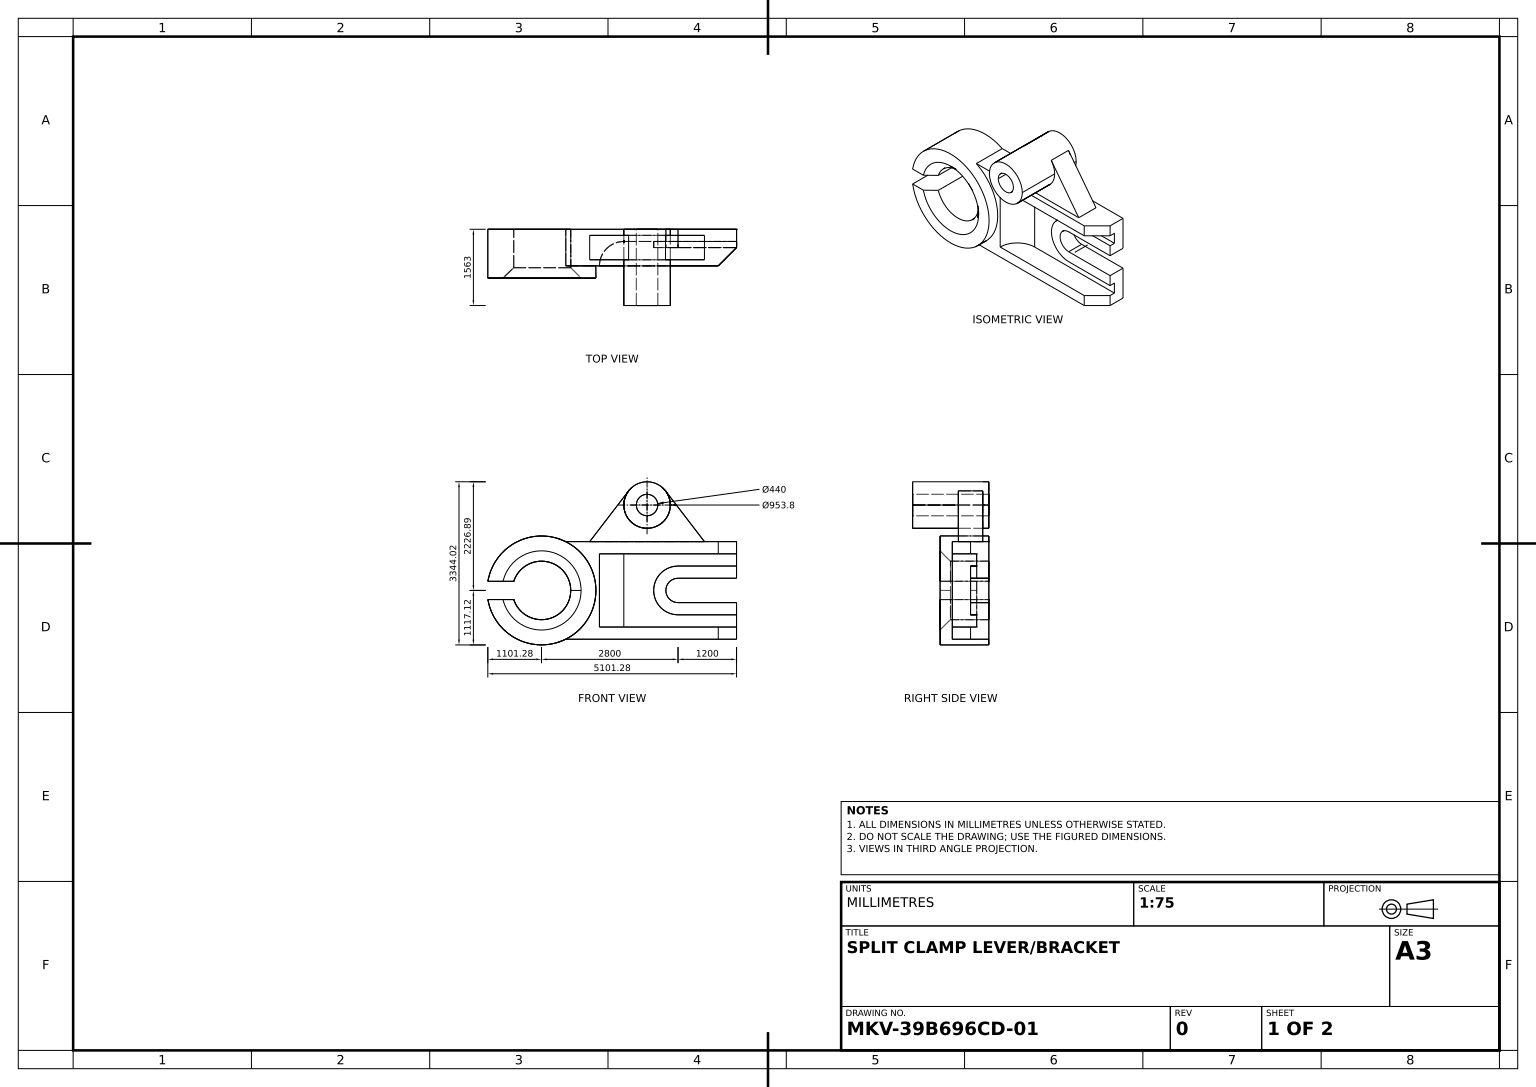
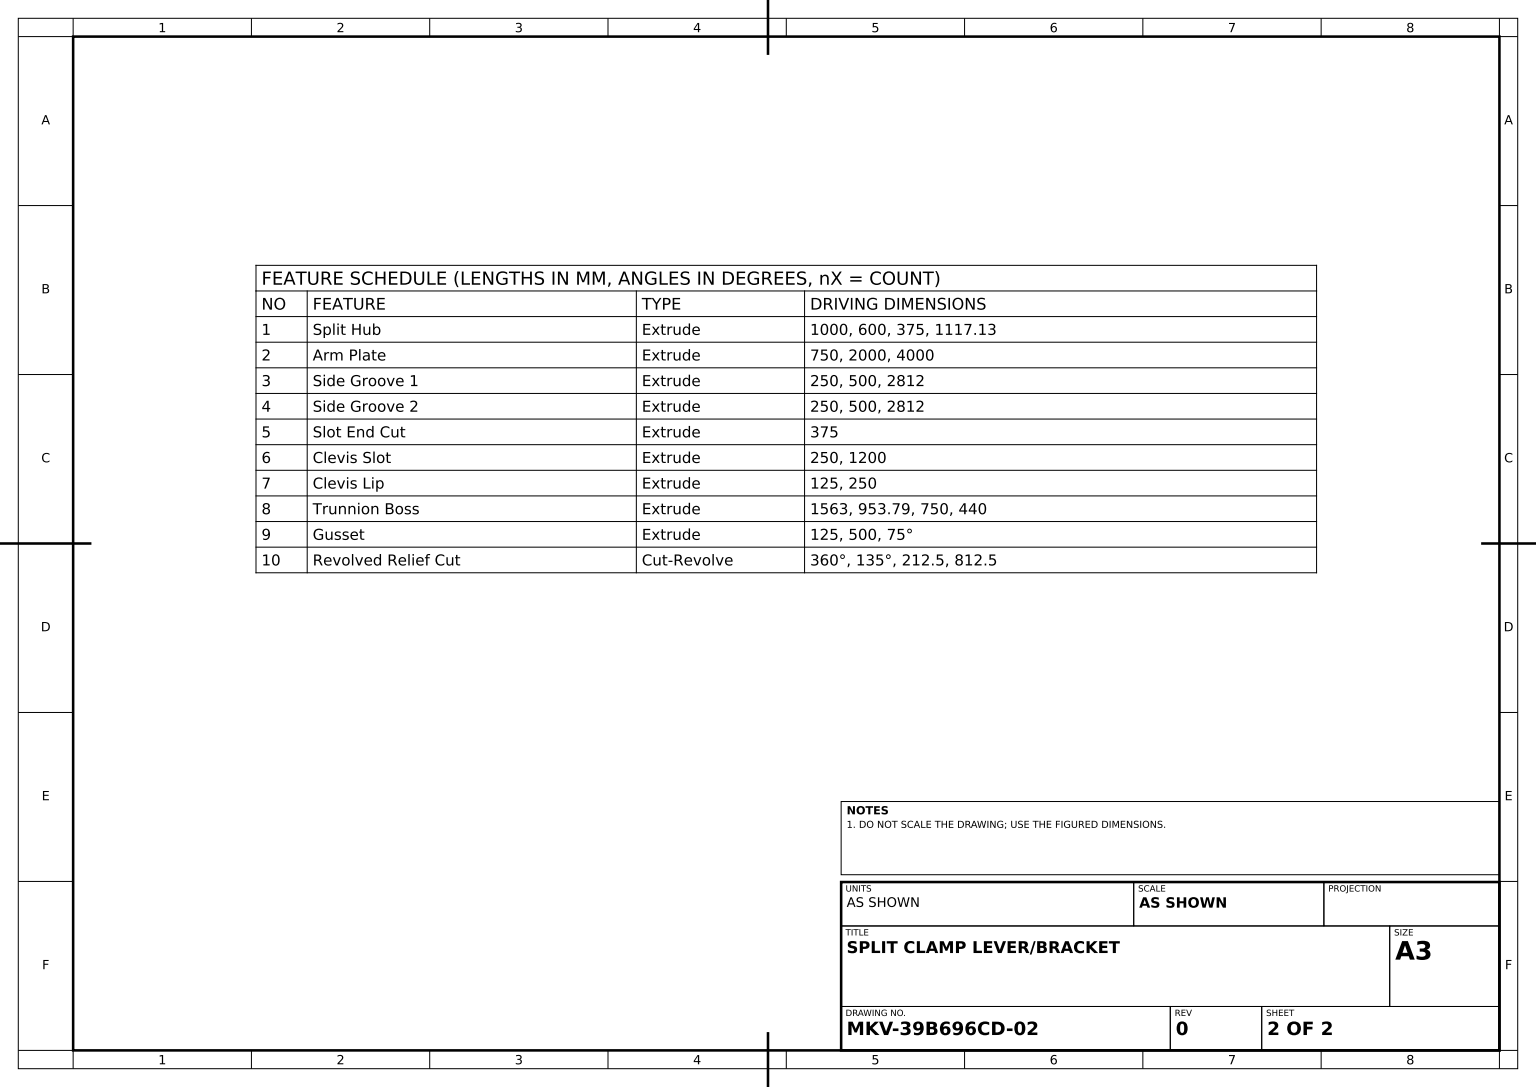
ISO-10303-21;
HEADER;
FILE_DESCRIPTION((''),'2;1');
FILE_NAME('','',(''),(''),'','','');
FILE_SCHEMA(('AUTOMOTIVE_DESIGN'));
ENDSEC;
DATA;
#1=APPLICATION_CONTEXT('');
#2=PRODUCT_CONTEXT('',#1,'mechanical');
#3=PRODUCT('','','',(#2));
#4=PRODUCT_DEFINITION_FORMATION('','',#3);
#5=PRODUCT_DEFINITION_CONTEXT('',#1,'design');
#6=PRODUCT_DEFINITION('','',#4,#5);
#7=PRODUCT_DEFINITION_SHAPE('','',#6);
#8=(LENGTH_UNIT()NAMED_UNIT(*)SI_UNIT(.MILLI.,.METRE.));
#9=(NAMED_UNIT(*)PLANE_ANGLE_UNIT()SI_UNIT($,.RADIAN.));
#10=(NAMED_UNIT(*)SI_UNIT($,.STERADIAN.)SOLID_ANGLE_UNIT());
#11=UNCERTAINTY_MEASURE_WITH_UNIT(LENGTH_MEASURE(1.E-05),#8,'distance_accuracy_value','');
#12=(GEOMETRIC_REPRESENTATION_CONTEXT(3)GLOBAL_UNCERTAINTY_ASSIGNED_CONTEXT((#11))GLOBAL_UNIT_ASSIGNED_CONTEXT((#8,#9,#10))REPRESENTATION_CONTEXT('',''));
#13=CARTESIAN_POINT('',(4000.,750.,250.));
#14=VERTEX_POINT('',#13);
#15=CARTESIAN_POINT('',(4000.,750.,375.));
#16=VERTEX_POINT('',#15);
#17=CARTESIAN_POINT('',(4000.,750.,750.));
#18=DIRECTION('',(0.,0.,1.));
#19=VECTOR('',#18,1000.);
#20=LINE('',#17,#19);
#21=EDGE_CURVE('',#14,#16,#20,.T.);
#22=ORIENTED_EDGE('',*,*,#21,.F.);
#23=CARTESIAN_POINT('',(4000.,500.,250.));
#24=VERTEX_POINT('',#23);
#25=CARTESIAN_POINT('',(4000.,3856.106441,250.));
#26=DIRECTION('',(0.,-1.,0.));
#27=VECTOR('',#26,1000.);
#28=LINE('',#25,#27);
#29=EDGE_CURVE('',#14,#24,#28,.T.);
#30=ORIENTED_EDGE('',*,*,#29,.T.);
#31=CARTESIAN_POINT('',(4000.,500.,375.));
#32=VERTEX_POINT('',#31);
#33=DIRECTION('',(0.,0.,-1.));
#34=VECTOR('',#33,1000.);
#35=LINE('',#31,#34);
#36=EDGE_CURVE('',#32,#24,#35,.T.);
#37=ORIENTED_EDGE('',*,*,#36,.F.);
#38=CARTESIAN_POINT('',(4000.,250.,375.));
#39=VERTEX_POINT('',#38);
#40=DIRECTION('',(0.,1.,0.));
#41=VECTOR('',#40,1000.);
#42=LINE('',#31,#41);
#43=EDGE_CURVE('',#39,#32,#42,.T.);
#44=ORIENTED_EDGE('',*,*,#43,.F.);
#45=CARTESIAN_POINT('',(4000.,250.,0.));
#46=VERTEX_POINT('',#45);
#47=LINE('',#45,#19);
#48=EDGE_CURVE('',#46,#39,#47,.T.);
#49=ORIENTED_EDGE('',*,*,#48,.F.);
#50=CARTESIAN_POINT('',(4000.,1000.,0.));
#51=VERTEX_POINT('',#50);
#52=LINE('',#50,#41);
#53=EDGE_CURVE('',#46,#51,#52,.T.);
#54=ORIENTED_EDGE('',*,*,#53,.T.);
#55=CARTESIAN_POINT('',(4000.,1000.,375.));
#56=VERTEX_POINT('',#55);
#57=CARTESIAN_POINT('',(4000.,1000.,750.));
#58=LINE('',#57,#34);
#59=EDGE_CURVE('',#56,#51,#58,.T.);
#60=ORIENTED_EDGE('',*,*,#59,.F.);
#61=CARTESIAN_POINT('',(4000.,-1117.13,375.));
#62=LINE('',#61,#41);
#63=EDGE_CURVE('',#16,#56,#62,.T.);
#64=ORIENTED_EDGE('',*,*,#63,.F.);
#65=EDGE_LOOP('',(#22,#30,#37,#44,#49,#54,#60,#64));
#66=FACE_OUTER_BOUND('',#65,.T.);
#67=DIRECTION('',(-1.,0.,0.));
#68=AXIS2_PLACEMENT_3D('',#57,#67,#18);
#69=PLANE('',#68);
#70=ADVANCED_FACE('',(#66),#69,.F.);
#71=CARTESIAN_POINT('',(3341.503233,1000.,625.));
#72=VERTEX_POINT('',#71);
#73=CARTESIAN_POINT('',(3341.503233,1000.,125.));
#74=VERTEX_POINT('',#73);
#75=LINE('',#71,#34);
#76=EDGE_CURVE('',#72,#74,#75,.T.);
#77=ORIENTED_EDGE('',*,*,#76,.T.);
#78=CARTESIAN_POINT('',(2543.241241,2040.315282,125.));
#79=VERTEX_POINT('',#78);
#80=DIRECTION('',(-0.608761429,0.79335334,0.));
#81=VECTOR('',#80,1000.);
#82=LINE('',#78,#81);
#83=EDGE_CURVE('',#74,#79,#82,.T.);
#84=ORIENTED_EDGE('',*,*,#83,.T.);
#85=CARTESIAN_POINT('',(2543.241241,2040.315282,625.));
#86=VERTEX_POINT('',#85);
#87=LINE('',#85,#34);
#88=EDGE_CURVE('',#86,#79,#87,.T.);
#89=ORIENTED_EDGE('',*,*,#88,.F.);
#90=LINE('',#85,#81);
#91=EDGE_CURVE('',#72,#86,#90,.T.);
#92=ORIENTED_EDGE('',*,*,#91,.F.);
#93=EDGE_LOOP('',(#77,#84,#89,#92));
#94=FACE_OUTER_BOUND('',#93,.T.);
#95=DIRECTION('',(-0.79335334,-0.608761429,0.));
#96=DIRECTION('',(0.608761429,-0.79335334,0.));
#97=AXIS2_PLACEMENT_3D('',#85,#95,#96);
#98=PLANE('',#97);
#99=ADVANCED_FACE('',(#94),#98,.F.);
#100=CARTESIAN_POINT('',(2300.,0.,250.));
#101=VERTEX_POINT('',#100);
#102=CARTESIAN_POINT('',(2800.,-500.,250.));
#103=VERTEX_POINT('',#102);
#104=CARTESIAN_POINT('',(2800.,0.,250.));
#105=DIRECTION('',(1.,0.,0.));
#106=AXIS2_PLACEMENT_3D('',#104,#18,#105);
#107=CIRCLE('',#106,500.);
#108=EDGE_CURVE('',#101,#103,#107,.T.);
#109=ORIENTED_EDGE('',*,*,#108,.T.);
#110=CARTESIAN_POINT('',(2800.,-500.,375.));
#111=VERTEX_POINT('',#110);
#112=LINE('',#110,#34);
#113=EDGE_CURVE('',#111,#103,#112,.T.);
#114=ORIENTED_EDGE('',*,*,#113,.F.);
#115=CARTESIAN_POINT('',(2300.,0.,375.));
#116=VERTEX_POINT('',#115);
#117=CARTESIAN_POINT('',(2800.,0.,375.));
#118=AXIS2_PLACEMENT_3D('',#117,#18,#105);
#119=CIRCLE('',#118,500.);
#120=EDGE_CURVE('',#116,#111,#119,.T.);
#121=ORIENTED_EDGE('',*,*,#120,.F.);
#122=LINE('',#115,#34);
#123=EDGE_CURVE('',#116,#101,#122,.T.);
#124=ORIENTED_EDGE('',*,*,#123,.T.);
#125=EDGE_LOOP('',(#109,#114,#121,#124));
#126=FACE_OUTER_BOUND('',#125,.T.);
#127=AXIS2_PLACEMENT_3D('',#117,#33,#67);
#128=CYLINDRICAL_SURFACE('',#127,500.);
#129=ADVANCED_FACE('',(#126),#128,.T.);
#130=CARTESIAN_POINT('',(1786.548759,2040.315282,625.));
#131=VERTEX_POINT('',#130);
#132=CARTESIAN_POINT('',(1786.548759,2040.315282,125.));
#133=VERTEX_POINT('',#132);
#134=LINE('',#130,#34);
#135=EDGE_CURVE('',#131,#133,#134,.T.);
#136=ORIENTED_EDGE('',*,*,#135,.T.);
#137=CARTESIAN_POINT('',(988.286767,1000.,125.));
#138=VERTEX_POINT('',#137);
#139=DIRECTION('',(-0.608761429,-0.79335334,0.));
#140=VECTOR('',#139,1000.);
#141=LINE('',#132,#140);
#142=EDGE_CURVE('',#133,#138,#141,.T.);
#143=ORIENTED_EDGE('',*,*,#142,.T.);
#144=CARTESIAN_POINT('',(988.286767,1000.,625.));
#145=VERTEX_POINT('',#144);
#146=LINE('',#144,#34);
#147=EDGE_CURVE('',#145,#138,#146,.T.);
#148=ORIENTED_EDGE('',*,*,#147,.F.);
#149=LINE('',#130,#140);
#150=EDGE_CURVE('',#131,#145,#149,.T.);
#151=ORIENTED_EDGE('',*,*,#150,.F.);
#152=EDGE_LOOP('',(#136,#143,#148,#151));
#153=FACE_OUTER_BOUND('',#152,.T.);
#154=DIRECTION('',(0.79335334,-0.608761429,0.));
#155=DIRECTION('',(0.608761429,0.79335334,0.));
#156=AXIS2_PLACEMENT_3D('',#130,#154,#155);
#157=PLANE('',#156);
#158=ADVANCED_FACE('',(#153),#157,.F.);
#159=CARTESIAN_POINT('',(2384.895,1750.,1563.));
#160=VERTEX_POINT('',#159);
#161=CARTESIAN_POINT('',(1944.895,1750.,1563.));
#162=VERTEX_POINT('',#161);
#163=CARTESIAN_POINT('',(2164.895,1750.,1563.));
#164=AXIS2_PLACEMENT_3D('',#163,#33,#67);
#165=CIRCLE('',#164,220.);
#166=EDGE_CURVE('',#160,#162,#165,.T.);
#167=ORIENTED_EDGE('',*,*,#166,.T.);
#168=EDGE_CURVE('',#162,#160,#165,.T.);
#169=ORIENTED_EDGE('',*,*,#168,.T.);
#170=EDGE_LOOP('',(#167,#169));
#171=FACE_BOUND('',#170,.T.);
#172=CARTESIAN_POINT('',(2641.79,1750.,1563.));
#173=VERTEX_POINT('',#172);
#174=CARTESIAN_POINT('',(1688.,1750.,1563.));
#175=VERTEX_POINT('',#174);
#176=CIRCLE('',#164,476.895);
#177=EDGE_CURVE('',#173,#175,#176,.T.);
#178=ORIENTED_EDGE('',*,*,#177,.F.);
#179=EDGE_CURVE('',#175,#173,#176,.T.);
#180=ORIENTED_EDGE('',*,*,#179,.F.);
#181=EDGE_LOOP('',(#178,#180));
#182=FACE_OUTER_BOUND('',#181,.T.);
#183=PLANE('',#164);
#184=ADVANCED_FACE('',(#171,#182),#183,.F.);
#185=CARTESIAN_POINT('',(1188.,750.,750.));
#186=VERTEX_POINT('',#185);
#187=CARTESIAN_POINT('',(1188.,-750.,750.));
#188=VERTEX_POINT('',#187);
#189=CARTESIAN_POINT('',(1188.,3856.106441,750.));
#190=LINE('',#189,#27);
#191=EDGE_CURVE('',#186,#188,#190,.T.);
#192=ORIENTED_EDGE('',*,*,#191,.T.);
#193=CARTESIAN_POINT('',(1688.,-750.,250.));
#194=VERTEX_POINT('',#193);
#195=CARTESIAN_POINT('',(1688.,-750.,750.));
#196=AXIS2_PLACEMENT_3D('',#195,#26,#67);
#197=CIRCLE('',#196,500.);
#198=EDGE_CURVE('',#188,#194,#197,.T.);
#199=ORIENTED_EDGE('',*,*,#198,.T.);
#200=CARTESIAN_POINT('',(1688.,750.,250.));
#201=VERTEX_POINT('',#200);
#202=CARTESIAN_POINT('',(1688.,3856.106441,250.));
#203=LINE('',#202,#27);
#204=EDGE_CURVE('',#201,#194,#203,.T.);
#205=ORIENTED_EDGE('',*,*,#204,.F.);
#206=CARTESIAN_POINT('',(1688.,750.,750.));
#207=AXIS2_PLACEMENT_3D('',#206,#26,#105);
#208=CIRCLE('',#207,500.);
#209=EDGE_CURVE('',#186,#201,#208,.T.);
#210=ORIENTED_EDGE('',*,*,#209,.F.);
#211=EDGE_LOOP('',(#192,#199,#205,#210));
#212=FACE_OUTER_BOUND('',#211,.T.);
#213=CARTESIAN_POINT('',(1688.,3856.106441,750.));
#214=AXIS2_PLACEMENT_3D('',#213,#26,#33);
#215=CYLINDRICAL_SURFACE('',#214,500.);
#216=ADVANCED_FACE('',(#212),#215,.F.);
#217=CARTESIAN_POINT('',(4000.,-500.,250.));
#218=VERTEX_POINT('',#217);
#219=VECTOR('',#105,1000.);
#220=LINE('',#102,#219);
#221=EDGE_CURVE('',#103,#218,#220,.T.);
#222=ORIENTED_EDGE('',*,*,#221,.T.);
#223=CARTESIAN_POINT('',(4000.,-500.,375.));
#224=VERTEX_POINT('',#223);
#225=LINE('',#223,#34);
#226=EDGE_CURVE('',#224,#218,#225,.T.);
#227=ORIENTED_EDGE('',*,*,#226,.F.);
#228=LINE('',#110,#219);
#229=EDGE_CURVE('',#111,#224,#228,.T.);
#230=ORIENTED_EDGE('',*,*,#229,.F.);
#231=ORIENTED_EDGE('',*,*,#113,.T.);
#232=EDGE_LOOP('',(#222,#227,#230,#231));
#233=FACE_OUTER_BOUND('',#232,.T.);
#234=AXIS2_PLACEMENT_3D('',#110,#40,#18);
#235=PLANE('',#234);
#236=ADVANCED_FACE('',(#233),#235,.F.);
#237=CARTESIAN_POINT('',(2800.,500.,250.));
#238=VERTEX_POINT('',#237);
#239=EDGE_CURVE('',#238,#101,#107,.T.);
#240=ORIENTED_EDGE('',*,*,#239,.T.);
#241=ORIENTED_EDGE('',*,*,#123,.F.);
#242=CARTESIAN_POINT('',(2800.,500.,375.));
#243=VERTEX_POINT('',#242);
#244=EDGE_CURVE('',#243,#116,#119,.T.);
#245=ORIENTED_EDGE('',*,*,#244,.F.);
#246=LINE('',#242,#34);
#247=EDGE_CURVE('',#243,#238,#246,.T.);
#248=ORIENTED_EDGE('',*,*,#247,.T.);
#249=EDGE_LOOP('',(#240,#241,#245,#248));
#250=FACE_OUTER_BOUND('',#249,.T.);
#251=ADVANCED_FACE('',(#250),#128,.T.);
#252=CARTESIAN_POINT('',(2384.895,1750.,0.));
#253=VERTEX_POINT('',#252);
#254=LINE('',#159,#34);
#255=EDGE_CURVE('',#160,#253,#254,.T.);
#256=ORIENTED_EDGE('',*,*,#255,.T.);
#257=CARTESIAN_POINT('',(1944.895,1750.,0.));
#258=VERTEX_POINT('',#257);
#259=CARTESIAN_POINT('',(2164.895,1750.,0.));
#260=AXIS2_PLACEMENT_3D('',#259,#33,#67);
#261=CIRCLE('',#260,220.);
#262=EDGE_CURVE('',#253,#258,#261,.T.);
#263=ORIENTED_EDGE('',*,*,#262,.T.);
#264=LINE('',#161,#34);
#265=EDGE_CURVE('',#162,#258,#264,.T.);
#266=ORIENTED_EDGE('',*,*,#265,.F.);
#267=ORIENTED_EDGE('',*,*,#166,.F.);
#268=EDGE_LOOP('',(#256,#263,#266,#267));
#269=FACE_OUTER_BOUND('',#268,.T.);
#270=CYLINDRICAL_SURFACE('',#164,220.);
#271=ADVANCED_FACE('',(#269),#270,.F.);
#272=CARTESIAN_POINT('',(-790.569415,-187.5,1000.));
#273=VERTEX_POINT('',#272);
#274=CARTESIAN_POINT('',(-1101.282519,-187.5,1000.));
#275=VERTEX_POINT('',#274);
#276=VECTOR('',#67,1000.);
#277=LINE('',#274,#276);
#278=EDGE_CURVE('',#273,#275,#277,.T.);
#279=ORIENTED_EDGE('',*,*,#278,.T.);
#280=CARTESIAN_POINT('',(-1101.282519,187.5,1000.));
#281=VERTEX_POINT('',#280);
#282=CARTESIAN_POINT('',(0.,0.,1000.));
#283=AXIS2_PLACEMENT_3D('',#282,#18,#105);
#284=CIRCLE('',#283,1117.13);
#285=EDGE_CURVE('',#275,#281,#284,.T.);
#286=ORIENTED_EDGE('',*,*,#285,.T.);
#287=CARTESIAN_POINT('',(-790.569415,187.5,1000.));
#288=VERTEX_POINT('',#287);
#289=LINE('',#280,#219);
#290=EDGE_CURVE('',#281,#288,#289,.T.);
#291=ORIENTED_EDGE('',*,*,#290,.T.);
#292=CARTESIAN_POINT('',(812.5,0.,1000.));
#293=VERTEX_POINT('',#292);
#294=AXIS2_PLACEMENT_3D('',#282,#33,#67);
#295=CIRCLE('',#294,812.5);
#296=EDGE_CURVE('',#288,#293,#295,.T.);
#297=ORIENTED_EDGE('',*,*,#296,.T.);
#298=EDGE_CURVE('',#293,#273,#295,.T.);
#299=ORIENTED_EDGE('',*,*,#298,.T.);
#300=EDGE_LOOP('',(#279,#286,#291,#297,#299));
#301=FACE_OUTER_BOUND('',#300,.T.);
#302=PLANE('',#283);
#303=ADVANCED_FACE('',(#301),#302,.T.);
#304=CARTESIAN_POINT('',(2800.,-250.,0.));
#305=VERTEX_POINT('',#304);
#306=CARTESIAN_POINT('',(2800.,-250.,375.));
#307=VERTEX_POINT('',#306);
#308=LINE('',#304,#19);
#309=EDGE_CURVE('',#305,#307,#308,.T.);
#310=ORIENTED_EDGE('',*,*,#309,.F.);
#311=CARTESIAN_POINT('',(2800.,250.,0.));
#312=VERTEX_POINT('',#311);
#313=CARTESIAN_POINT('',(2800.,0.,0.));
#314=AXIS2_PLACEMENT_3D('',#313,#18,#67);
#315=CIRCLE('',#314,250.);
#316=EDGE_CURVE('',#312,#305,#315,.T.);
#317=ORIENTED_EDGE('',*,*,#316,.F.);
#318=CARTESIAN_POINT('',(2800.,250.,375.));
#319=VERTEX_POINT('',#318);
#320=LINE('',#311,#19);
#321=EDGE_CURVE('',#312,#319,#320,.T.);
#322=ORIENTED_EDGE('',*,*,#321,.T.);
#323=AXIS2_PLACEMENT_3D('',#117,#33,#105);
#324=CIRCLE('',#323,250.);
#325=EDGE_CURVE('',#307,#319,#324,.T.);
#326=ORIENTED_EDGE('',*,*,#325,.F.);
#327=EDGE_LOOP('',(#310,#317,#322,#326));
#328=FACE_OUTER_BOUND('',#327,.T.);
#329=AXIS2_PLACEMENT_3D('',#313,#18,#105);
#330=CYLINDRICAL_SURFACE('',#329,250.);
#331=ADVANCED_FACE('',(#328),#330,.F.);
#332=ORIENTED_EDGE('',*,*,#247,.F.);
#333=LINE('',#242,#276);
#334=EDGE_CURVE('',#32,#243,#333,.T.);
#335=ORIENTED_EDGE('',*,*,#334,.F.);
#336=ORIENTED_EDGE('',*,*,#36,.T.);
#337=LINE('',#237,#276);
#338=EDGE_CURVE('',#24,#238,#337,.T.);
#339=ORIENTED_EDGE('',*,*,#338,.T.);
#340=EDGE_LOOP('',(#332,#335,#336,#339));
#341=FACE_OUTER_BOUND('',#340,.T.);
#342=AXIS2_PLACEMENT_3D('',#242,#26,#33);
#343=PLANE('',#342);
#344=ADVANCED_FACE('',(#341),#343,.F.);
#345=CARTESIAN_POINT('',(497.975338,1000.,0.));
#346=VERTEX_POINT('',#345);
#347=CARTESIAN_POINT('',(-1101.282519,187.5,0.));
#348=VERTEX_POINT('',#347);
#349=CARTESIAN_POINT('',(0.,0.,0.));
#350=AXIS2_PLACEMENT_3D('',#349,#18,#105);
#351=CIRCLE('',#350,1117.13);
#352=EDGE_CURVE('',#346,#348,#351,.T.);
#353=ORIENTED_EDGE('',*,*,#352,.T.);
#354=LINE('',#280,#34);
#355=EDGE_CURVE('',#281,#348,#354,.T.);
#356=ORIENTED_EDGE('',*,*,#355,.F.);
#357=ORIENTED_EDGE('',*,*,#285,.F.);
#358=CARTESIAN_POINT('',(-1101.282519,-187.5,0.));
#359=VERTEX_POINT('',#358);
#360=LINE('',#274,#34);
#361=EDGE_CURVE('',#275,#359,#360,.T.);
#362=ORIENTED_EDGE('',*,*,#361,.T.);
#363=CARTESIAN_POINT('',(497.975338,-1000.,0.));
#364=VERTEX_POINT('',#363);
#365=EDGE_CURVE('',#359,#364,#351,.T.);
#366=ORIENTED_EDGE('',*,*,#365,.T.);
#367=CARTESIAN_POINT('',(497.975338,-1000.,750.));
#368=VERTEX_POINT('',#367);
#369=LINE('',#367,#34);
#370=EDGE_CURVE('',#368,#364,#369,.T.);
#371=ORIENTED_EDGE('',*,*,#370,.F.);
#372=CARTESIAN_POINT('',(497.975338,1000.,750.));
#373=VERTEX_POINT('',#372);
#374=CARTESIAN_POINT('',(0.,0.,750.));
#375=AXIS2_PLACEMENT_3D('',#374,#33,#105);
#376=CIRCLE('',#375,1117.13);
#377=EDGE_CURVE('',#373,#368,#376,.T.);
#378=ORIENTED_EDGE('',*,*,#377,.F.);
#379=LINE('',#372,#34);
#380=EDGE_CURVE('',#373,#346,#379,.T.);
#381=ORIENTED_EDGE('',*,*,#380,.T.);
#382=EDGE_LOOP('',(#353,#356,#357,#362,#366,#371,#378,#381));
#383=FACE_OUTER_BOUND('',#382,.T.);
#384=CYLINDRICAL_SURFACE('',#294,1117.13);
#385=ADVANCED_FACE('',(#383),#384,.T.);
#386=ORIENTED_EDGE('',*,*,#365,.F.);
#387=CARTESIAN_POINT('',(-569.950656,-187.5,0.));
#388=VERTEX_POINT('',#387);
#389=LINE('',#358,#276);
#390=EDGE_CURVE('',#388,#359,#389,.T.);
#391=ORIENTED_EDGE('',*,*,#390,.F.);
#392=CARTESIAN_POINT('',(-569.950656,187.5,0.));
#393=VERTEX_POINT('',#392);
#394=AXIS2_PLACEMENT_3D('',#349,#33,#105);
#395=CIRCLE('',#394,600.);
#396=EDGE_CURVE('',#393,#388,#395,.T.);
#397=ORIENTED_EDGE('',*,*,#396,.F.);
#398=LINE('',#347,#219);
#399=EDGE_CURVE('',#348,#393,#398,.T.);
#400=ORIENTED_EDGE('',*,*,#399,.F.);
#401=ORIENTED_EDGE('',*,*,#352,.F.);
#402=LINE('',#345,#276);
#403=EDGE_CURVE('',#51,#346,#402,.T.);
#404=ORIENTED_EDGE('',*,*,#403,.F.);
#405=ORIENTED_EDGE('',*,*,#53,.F.);
#406=LINE('',#311,#276);
#407=EDGE_CURVE('',#46,#312,#406,.T.);
#408=ORIENTED_EDGE('',*,*,#407,.T.);
#409=ORIENTED_EDGE('',*,*,#316,.T.);
#410=CARTESIAN_POINT('',(4000.,-250.,0.));
#411=VERTEX_POINT('',#410);
#412=LINE('',#410,#219);
#413=EDGE_CURVE('',#305,#411,#412,.T.);
#414=ORIENTED_EDGE('',*,*,#413,.T.);
#415=CARTESIAN_POINT('',(4000.,-1000.,0.));
#416=VERTEX_POINT('',#415);
#417=EDGE_CURVE('',#416,#411,#52,.T.);
#418=ORIENTED_EDGE('',*,*,#417,.F.);
#419=LINE('',#415,#219);
#420=EDGE_CURVE('',#364,#416,#419,.T.);
#421=ORIENTED_EDGE('',*,*,#420,.F.);
#422=EDGE_LOOP('',(#386,#391,#397,#400,#401,#404,#405,#408,#409,#414,#418,#421));
#423=FACE_OUTER_BOUND('',#422,.T.);
#424=PLANE('',#350);
#425=ADVANCED_FACE('',(#423),#424,.F.);
#426=CARTESIAN_POINT('',(1688.,1750.,625.));
#427=VERTEX_POINT('',#426);
#428=LINE('',#174,#34);
#429=EDGE_CURVE('',#175,#427,#428,.T.);
#430=ORIENTED_EDGE('',*,*,#429,.T.);
#431=CARTESIAN_POINT('',(2641.79,1750.,625.));
#432=VERTEX_POINT('',#431);
#433=CARTESIAN_POINT('',(2164.895,1750.,625.));
#434=AXIS2_PLACEMENT_3D('',#433,#33,#105);
#435=CIRCLE('',#434,476.895);
#436=EDGE_CURVE('',#432,#427,#435,.T.);
#437=ORIENTED_EDGE('',*,*,#436,.F.);
#438=LINE('',#172,#34);
#439=EDGE_CURVE('',#173,#432,#438,.T.);
#440=ORIENTED_EDGE('',*,*,#439,.F.);
#441=ORIENTED_EDGE('',*,*,#177,.T.);
#442=EDGE_LOOP('',(#430,#437,#440,#441));
#443=FACE_OUTER_BOUND('',#442,.T.);
#444=CYLINDRICAL_SURFACE('',#164,476.895);
#445=ADVANCED_FACE('',(#443),#444,.T.);
#446=LINE('',#137,#219);
#447=EDGE_CURVE('',#138,#74,#446,.T.);
#448=ORIENTED_EDGE('',*,*,#447,.T.);
#449=ORIENTED_EDGE('',*,*,#76,.F.);
#450=LINE('',#144,#219);
#451=EDGE_CURVE('',#145,#72,#450,.T.);
#452=ORIENTED_EDGE('',*,*,#451,.F.);
#453=ORIENTED_EDGE('',*,*,#147,.T.);
#454=EDGE_LOOP('',(#448,#449,#452,#453));
#455=FACE_BOUND('',#454,.T.);
#456=ORIENTED_EDGE('',*,*,#403,.T.);
#457=ORIENTED_EDGE('',*,*,#380,.F.);
#458=CARTESIAN_POINT('',(3625.,1000.,750.));
#459=VERTEX_POINT('',#458);
#460=LINE('',#372,#276);
#461=EDGE_CURVE('',#459,#373,#460,.T.);
#462=ORIENTED_EDGE('',*,*,#461,.F.);
#463=DIRECTION('',(-0.707106781,0.,0.707106781));
#464=VECTOR('',#463,1000.);
#465=LINE('',#55,#464);
#466=EDGE_CURVE('',#56,#459,#465,.T.);
#467=ORIENTED_EDGE('',*,*,#466,.F.);
#468=ORIENTED_EDGE('',*,*,#59,.T.);
#469=EDGE_LOOP('',(#456,#457,#462,#467,#468));
#470=FACE_OUTER_BOUND('',#469,.T.);
#471=AXIS2_PLACEMENT_3D('',#372,#26,#105);
#472=PLANE('',#471);
#473=ADVANCED_FACE('',(#455,#470),#472,.F.);
#474=ORIENTED_EDGE('',*,*,#361,.F.);
#475=ORIENTED_EDGE('',*,*,#278,.F.);
#476=CARTESIAN_POINT('',(-569.950656,-187.5,787.5));
#477=VERTEX_POINT('',#476);
#478=CARTESIAN_POINT('',(-753.977239,-187.5,964.395502));
#479=CARTESIAN_POINT('',(-717.321809,-187.5,928.857895));
#480=CARTESIAN_POINT('',(-662.191148,-187.5,875.707485));
#481=CARTESIAN_POINT('',(-643.789398,-187.5,858.016974));
#482=CARTESIAN_POINT('',(-606.922384,-187.5,822.703119));
#483=CARTESIAN_POINT('',(-588.457198,-187.5,805.079693));
#484=B_SPLINE_CURVE_WITH_KNOTS('',3,(#272,#478,#479,#480,#481,#482,#483,#476),.UNSPECIFIED.,.F.,.F.,(4,2,2,4),(0.460466118,0.613617143,0.690192656,0.766768169),.UNSPECIFIED.);
#485=EDGE_CURVE('',#273,#477,#484,.T.);
#486=ORIENTED_EDGE('',*,*,#485,.T.);
#487=CARTESIAN_POINT('',(-569.950656,-187.5,1000.));
#488=LINE('',#487,#34);
#489=EDGE_CURVE('',#477,#388,#488,.T.);
#490=ORIENTED_EDGE('',*,*,#489,.T.);
#491=ORIENTED_EDGE('',*,*,#390,.T.);
#492=EDGE_LOOP('',(#474,#475,#486,#490,#491));
#493=FACE_OUTER_BOUND('',#492,.T.);
#494=AXIS2_PLACEMENT_3D('',#274,#26,#105);
#495=PLANE('',#494);
#496=ADVANCED_FACE('',(#493),#495,.F.);
#497=CARTESIAN_POINT('',(3625.,-1000.,750.));
#498=VERTEX_POINT('',#497);
#499=CARTESIAN_POINT('',(3625.,-750.,750.));
#500=VERTEX_POINT('',#499);
#501=CARTESIAN_POINT('',(3625.,-1117.13,750.));
#502=LINE('',#501,#41);
#503=EDGE_CURVE('',#498,#500,#502,.T.);
#504=ORIENTED_EDGE('',*,*,#503,.T.);
#505=LINE('',#187,#276);
#506=EDGE_CURVE('',#500,#188,#505,.T.);
#507=ORIENTED_EDGE('',*,*,#506,.T.);
#508=ORIENTED_EDGE('',*,*,#191,.F.);
#509=CARTESIAN_POINT('',(3625.,750.,750.));
#510=VERTEX_POINT('',#509);
#511=LINE('',#185,#276);
#512=EDGE_CURVE('',#510,#186,#511,.T.);
#513=ORIENTED_EDGE('',*,*,#512,.F.);
#514=EDGE_CURVE('',#510,#459,#502,.T.);
#515=ORIENTED_EDGE('',*,*,#514,.T.);
#516=ORIENTED_EDGE('',*,*,#461,.T.);
#517=ORIENTED_EDGE('',*,*,#377,.T.);
#518=CARTESIAN_POINT('',(4000.,-1000.,750.));
#519=LINE('',#518,#219);
#520=EDGE_CURVE('',#368,#498,#519,.T.);
#521=ORIENTED_EDGE('',*,*,#520,.T.);
#522=EDGE_LOOP('',(#504,#507,#508,#513,#515,#516,#517,#521));
#523=FACE_OUTER_BOUND('',#522,.T.);
#524=AXIS2_PLACEMENT_3D('',#374,#18,#105);
#525=PLANE('',#524);
#526=ADVANCED_FACE('',(#523),#525,.T.);
#527=ORIENTED_EDGE('',*,*,#325,.T.);
#528=LINE('',#38,#219);
#529=EDGE_CURVE('',#319,#39,#528,.T.);
#530=ORIENTED_EDGE('',*,*,#529,.T.);
#531=ORIENTED_EDGE('',*,*,#43,.T.);
#532=ORIENTED_EDGE('',*,*,#334,.T.);
#533=ORIENTED_EDGE('',*,*,#244,.T.);
#534=ORIENTED_EDGE('',*,*,#120,.T.);
#535=ORIENTED_EDGE('',*,*,#229,.T.);
#536=CARTESIAN_POINT('',(4000.,-250.,375.));
#537=VERTEX_POINT('',#536);
#538=LINE('',#223,#41);
#539=EDGE_CURVE('',#224,#537,#538,.T.);
#540=ORIENTED_EDGE('',*,*,#539,.T.);
#541=LINE('',#306,#276);
#542=EDGE_CURVE('',#537,#307,#541,.T.);
#543=ORIENTED_EDGE('',*,*,#542,.T.);
#544=EDGE_LOOP('',(#527,#530,#531,#532,#533,#534,#535,#540,#543));
#545=FACE_OUTER_BOUND('',#544,.T.);
#546=PLANE('',#118);
#547=ADVANCED_FACE('',(#545),#546,.T.);
#548=LINE('',#13,#219);
#549=EDGE_CURVE('',#201,#14,#548,.T.);
#550=ORIENTED_EDGE('',*,*,#549,.T.);
#551=ORIENTED_EDGE('',*,*,#21,.T.);
#552=CARTESIAN_POINT('',(2061.487669,750.,2313.512331));
#553=DIRECTION('',(0.707106781,0.,-0.707106781));
#554=VECTOR('',#553,1000.);
#555=LINE('',#552,#554);
#556=EDGE_CURVE('',#510,#16,#555,.T.);
#557=ORIENTED_EDGE('',*,*,#556,.F.);
#558=ORIENTED_EDGE('',*,*,#512,.T.);
#559=ORIENTED_EDGE('',*,*,#209,.T.);
#560=EDGE_LOOP('',(#550,#551,#557,#558,#559));
#561=FACE_OUTER_BOUND('',#560,.T.);
#562=CARTESIAN_POINT('',(497.975338,750.,750.));
#563=AXIS2_PLACEMENT_3D('',#562,#26,#105);
#564=PLANE('',#563);
#565=ADVANCED_FACE('',(#561),#564,.T.);
#566=CARTESIAN_POINT('',(4000.,-1000.,375.));
#567=VERTEX_POINT('',#566);
#568=LINE('',#518,#34);
#569=EDGE_CURVE('',#567,#416,#568,.T.);
#570=ORIENTED_EDGE('',*,*,#569,.F.);
#571=CARTESIAN_POINT('',(3812.5,-1000.,562.5));
#572=LINE('',#571,#464);
#573=EDGE_CURVE('',#567,#498,#572,.T.);
#574=ORIENTED_EDGE('',*,*,#573,.T.);
#575=ORIENTED_EDGE('',*,*,#520,.F.);
#576=ORIENTED_EDGE('',*,*,#370,.T.);
#577=ORIENTED_EDGE('',*,*,#420,.T.);
#578=EDGE_LOOP('',(#570,#574,#575,#576,#577));
#579=FACE_OUTER_BOUND('',#578,.T.);
#580=AXIS2_PLACEMENT_3D('',#518,#40,#67);
#581=PLANE('',#580);
#582=ADVANCED_FACE('',(#579),#581,.F.);
#583=CARTESIAN_POINT('',(600.,0.,787.5));
#584=VERTEX_POINT('',#583);
#585=DIRECTION('',(0.707106781,0.,0.707106781));
#586=VECTOR('',#585,1000.);
#587=LINE('',#583,#586);
#588=EDGE_CURVE('',#584,#293,#587,.T.);
#589=ORIENTED_EDGE('',*,*,#588,.F.);
#590=CARTESIAN_POINT('',(0.,0.,787.5));
#591=AXIS2_PLACEMENT_3D('',#590,#33,#67);
#592=CIRCLE('',#591,600.);
#593=EDGE_CURVE('',#584,#477,#592,.T.);
#594=ORIENTED_EDGE('',*,*,#593,.T.);
#595=ORIENTED_EDGE('',*,*,#485,.F.);
#596=ORIENTED_EDGE('',*,*,#298,.F.);
#597=EDGE_LOOP('',(#589,#594,#595,#596));
#598=FACE_OUTER_BOUND('',#597,.T.);
#599=AXIS2_PLACEMENT_3D('',#590,#18,#105);
#600=CONICAL_SURFACE('',#599,600.,0.785398163);
#601=ADVANCED_FACE('',(#598),#600,.F.);
#602=ORIENTED_EDGE('',*,*,#436,.T.);
#603=EDGE_CURVE('',#427,#131,#435,.T.);
#604=ORIENTED_EDGE('',*,*,#603,.T.);
#605=ORIENTED_EDGE('',*,*,#150,.T.);
#606=ORIENTED_EDGE('',*,*,#451,.T.);
#607=ORIENTED_EDGE('',*,*,#91,.T.);
#608=EDGE_CURVE('',#86,#432,#435,.T.);
#609=ORIENTED_EDGE('',*,*,#608,.T.);
#610=EDGE_LOOP('',(#602,#604,#605,#606,#607,#609));
#611=FACE_OUTER_BOUND('',#610,.T.);
#612=AXIS2_PLACEMENT_3D('',#433,#18,#105);
#613=PLANE('',#612);
#614=ADVANCED_FACE('',(#611),#613,.T.);
#615=ORIENTED_EDGE('',*,*,#588,.T.);
#616=ORIENTED_EDGE('',*,*,#296,.F.);
#617=CARTESIAN_POINT('',(-569.950656,187.5,787.5));
#618=VERTEX_POINT('',#617);
#619=CARTESIAN_POINT('',(-588.458918,187.5,805.081327));
#620=CARTESIAN_POINT('',(-606.925232,187.5,822.705839));
#621=CARTESIAN_POINT('',(-643.793607,187.5,858.021014));
#622=CARTESIAN_POINT('',(-662.195589,187.5,875.711758));
#623=CARTESIAN_POINT('',(-717.325901,187.5,928.861855));
#624=CARTESIAN_POINT('',(-753.979722,187.5,964.397917));
#625=B_SPLINE_CURVE_WITH_KNOTS('',3,(#617,#619,#620,#621,#622,#623,#624,#287),.UNSPECIFIED.,.F.,.F.,(4,2,2,4),(0.433365497,0.509923117,0.586480738,0.739595979),.UNSPECIFIED.);
#626=EDGE_CURVE('',#618,#288,#625,.T.);
#627=ORIENTED_EDGE('',*,*,#626,.F.);
#628=EDGE_CURVE('',#618,#584,#592,.T.);
#629=ORIENTED_EDGE('',*,*,#628,.T.);
#630=EDGE_LOOP('',(#615,#616,#627,#629));
#631=FACE_OUTER_BOUND('',#630,.T.);
#632=ADVANCED_FACE('',(#631),#600,.F.);
#633=LINE('',#410,#19);
#634=EDGE_CURVE('',#411,#537,#633,.T.);
#635=ORIENTED_EDGE('',*,*,#634,.T.);
#636=ORIENTED_EDGE('',*,*,#539,.F.);
#637=ORIENTED_EDGE('',*,*,#226,.T.);
#638=CARTESIAN_POINT('',(4000.,-750.,250.));
#639=VERTEX_POINT('',#638);
#640=EDGE_CURVE('',#218,#639,#28,.T.);
#641=ORIENTED_EDGE('',*,*,#640,.T.);
#642=CARTESIAN_POINT('',(4000.,-750.,375.));
#643=VERTEX_POINT('',#642);
#644=CARTESIAN_POINT('',(4000.,-750.,750.));
#645=LINE('',#644,#19);
#646=EDGE_CURVE('',#639,#643,#645,.T.);
#647=ORIENTED_EDGE('',*,*,#646,.T.);
#648=EDGE_CURVE('',#567,#643,#62,.T.);
#649=ORIENTED_EDGE('',*,*,#648,.F.);
#650=ORIENTED_EDGE('',*,*,#569,.T.);
#651=ORIENTED_EDGE('',*,*,#417,.T.);
#652=EDGE_LOOP('',(#635,#636,#637,#641,#647,#649,#650,#651));
#653=FACE_OUTER_BOUND('',#652,.T.);
#654=ADVANCED_FACE('',(#653),#69,.F.);
#655=ORIENTED_EDGE('',*,*,#626,.T.);
#656=ORIENTED_EDGE('',*,*,#290,.F.);
#657=ORIENTED_EDGE('',*,*,#355,.T.);
#658=ORIENTED_EDGE('',*,*,#399,.T.);
#659=CARTESIAN_POINT('',(-569.950656,187.5,1000.));
#660=LINE('',#659,#34);
#661=EDGE_CURVE('',#618,#393,#660,.T.);
#662=ORIENTED_EDGE('',*,*,#661,.F.);
#663=EDGE_LOOP('',(#655,#656,#657,#658,#662));
#664=FACE_OUTER_BOUND('',#663,.T.);
#665=AXIS2_PLACEMENT_3D('',#280,#40,#67);
#666=PLANE('',#665);
#667=ADVANCED_FACE('',(#664),#666,.F.);
#668=ORIENTED_EDGE('',*,*,#573,.F.);
#669=ORIENTED_EDGE('',*,*,#648,.T.);
#670=CARTESIAN_POINT('',(3812.5,-750.,562.5));
#671=LINE('',#670,#464);
#672=EDGE_CURVE('',#643,#500,#671,.T.);
#673=ORIENTED_EDGE('',*,*,#672,.T.);
#674=ORIENTED_EDGE('',*,*,#503,.F.);
#675=EDGE_LOOP('',(#668,#669,#673,#674));
#676=FACE_OUTER_BOUND('',#675,.T.);
#677=DIRECTION('',(-0.707106781,0.,-0.707106781));
#678=AXIS2_PLACEMENT_3D('',#61,#677,#463);
#679=PLANE('',#678);
#680=ADVANCED_FACE('',(#676),#679,.F.);
#681=ORIENTED_EDGE('',*,*,#514,.F.);
#682=ORIENTED_EDGE('',*,*,#556,.T.);
#683=ORIENTED_EDGE('',*,*,#63,.T.);
#684=ORIENTED_EDGE('',*,*,#466,.T.);
#685=EDGE_LOOP('',(#681,#682,#683,#684));
#686=FACE_OUTER_BOUND('',#685,.T.);
#687=ADVANCED_FACE('',(#686),#679,.F.);
#688=CARTESIAN_POINT('',(2641.79,1750.,125.));
#689=VERTEX_POINT('',#688);
#690=CARTESIAN_POINT('',(1688.,1750.,125.));
#691=VERTEX_POINT('',#690);
#692=CARTESIAN_POINT('',(2164.895,1750.,125.));
#693=AXIS2_PLACEMENT_3D('',#692,#33,#105);
#694=CIRCLE('',#693,476.895);
#695=EDGE_CURVE('',#689,#691,#694,.T.);
#696=ORIENTED_EDGE('',*,*,#695,.T.);
#697=CARTESIAN_POINT('',(1688.,1750.,0.));
#698=VERTEX_POINT('',#697);
#699=EDGE_CURVE('',#691,#698,#428,.T.);
#700=ORIENTED_EDGE('',*,*,#699,.T.);
#701=CARTESIAN_POINT('',(2641.79,1750.,0.));
#702=VERTEX_POINT('',#701);
#703=CIRCLE('',#260,476.895);
#704=EDGE_CURVE('',#702,#698,#703,.T.);
#705=ORIENTED_EDGE('',*,*,#704,.F.);
#706=EDGE_CURVE('',#689,#702,#438,.T.);
#707=ORIENTED_EDGE('',*,*,#706,.F.);
#708=EDGE_LOOP('',(#696,#700,#705,#707));
#709=FACE_OUTER_BOUND('',#708,.T.);
#710=ADVANCED_FACE('',(#709),#444,.T.);
#711=ORIENTED_EDGE('',*,*,#542,.F.);
#712=ORIENTED_EDGE('',*,*,#634,.F.);
#713=ORIENTED_EDGE('',*,*,#413,.F.);
#714=ORIENTED_EDGE('',*,*,#309,.T.);
#715=EDGE_LOOP('',(#711,#712,#713,#714));
#716=FACE_OUTER_BOUND('',#715,.T.);
#717=AXIS2_PLACEMENT_3D('',#410,#26,#105);
#718=PLANE('',#717);
#719=ADVANCED_FACE('',(#716),#718,.F.);
#720=ORIENTED_EDGE('',*,*,#396,.T.);
#721=ORIENTED_EDGE('',*,*,#489,.F.);
#722=ORIENTED_EDGE('',*,*,#593,.F.);
#723=ORIENTED_EDGE('',*,*,#628,.F.);
#724=ORIENTED_EDGE('',*,*,#661,.T.);
#725=EDGE_LOOP('',(#720,#721,#722,#723,#724));
#726=FACE_OUTER_BOUND('',#725,.T.);
#727=CYLINDRICAL_SURFACE('',#294,600.);
#728=ADVANCED_FACE('',(#726),#727,.F.);
#729=ORIENTED_EDGE('',*,*,#646,.F.);
#730=LINE('',#638,#219);
#731=EDGE_CURVE('',#194,#639,#730,.T.);
#732=ORIENTED_EDGE('',*,*,#731,.F.);
#733=ORIENTED_EDGE('',*,*,#198,.F.);
#734=ORIENTED_EDGE('',*,*,#506,.F.);
#735=ORIENTED_EDGE('',*,*,#672,.F.);
#736=EDGE_LOOP('',(#729,#732,#733,#734,#735));
#737=FACE_OUTER_BOUND('',#736,.T.);
#738=AXIS2_PLACEMENT_3D('',#644,#40,#67);
#739=PLANE('',#738);
#740=ADVANCED_FACE('',(#737),#739,.T.);
#741=EDGE_CURVE('',#258,#253,#261,.T.);
#742=ORIENTED_EDGE('',*,*,#741,.F.);
#743=ORIENTED_EDGE('',*,*,#262,.F.);
#744=EDGE_LOOP('',(#742,#743));
#745=FACE_BOUND('',#744,.T.);
#746=ORIENTED_EDGE('',*,*,#704,.T.);
#747=EDGE_CURVE('',#698,#702,#703,.T.);
#748=ORIENTED_EDGE('',*,*,#747,.T.);
#749=EDGE_LOOP('',(#746,#748));
#750=FACE_OUTER_BOUND('',#749,.T.);
#751=PLANE('',#260);
#752=ADVANCED_FACE('',(#745,#750),#751,.T.);
#753=ORIENTED_EDGE('',*,*,#255,.F.);
#754=ORIENTED_EDGE('',*,*,#168,.F.);
#755=ORIENTED_EDGE('',*,*,#265,.T.);
#756=ORIENTED_EDGE('',*,*,#741,.T.);
#757=EDGE_LOOP('',(#753,#754,#755,#756));
#758=FACE_OUTER_BOUND('',#757,.T.);
#759=ADVANCED_FACE('',(#758),#270,.F.);
#760=ORIENTED_EDGE('',*,*,#731,.T.);
#761=ORIENTED_EDGE('',*,*,#640,.F.);
#762=ORIENTED_EDGE('',*,*,#221,.F.);
#763=ORIENTED_EDGE('',*,*,#108,.F.);
#764=ORIENTED_EDGE('',*,*,#239,.F.);
#765=ORIENTED_EDGE('',*,*,#338,.F.);
#766=ORIENTED_EDGE('',*,*,#29,.F.);
#767=ORIENTED_EDGE('',*,*,#549,.F.);
#768=ORIENTED_EDGE('',*,*,#204,.T.);
#769=EDGE_LOOP('',(#760,#761,#762,#763,#764,#765,#766,#767,#768));
#770=FACE_OUTER_BOUND('',#769,.T.);
#771=AXIS2_PLACEMENT_3D('',#25,#18,#105);
#772=PLANE('',#771);
#773=ADVANCED_FACE('',(#770),#772,.T.);
#774=ORIENTED_EDGE('',*,*,#83,.F.);
#775=ORIENTED_EDGE('',*,*,#447,.F.);
#776=ORIENTED_EDGE('',*,*,#142,.F.);
#777=EDGE_CURVE('',#691,#133,#694,.T.);
#778=ORIENTED_EDGE('',*,*,#777,.F.);
#779=ORIENTED_EDGE('',*,*,#695,.F.);
#780=EDGE_CURVE('',#79,#689,#694,.T.);
#781=ORIENTED_EDGE('',*,*,#780,.F.);
#782=EDGE_LOOP('',(#774,#775,#776,#778,#779,#781));
#783=FACE_OUTER_BOUND('',#782,.T.);
#784=AXIS2_PLACEMENT_3D('',#692,#18,#105);
#785=PLANE('',#784);
#786=ADVANCED_FACE('',(#783),#785,.F.);
#787=ORIENTED_EDGE('',*,*,#48,.T.);
#788=ORIENTED_EDGE('',*,*,#529,.F.);
#789=ORIENTED_EDGE('',*,*,#321,.F.);
#790=ORIENTED_EDGE('',*,*,#407,.F.);
#791=EDGE_LOOP('',(#787,#788,#789,#790));
#792=FACE_OUTER_BOUND('',#791,.T.);
#793=AXIS2_PLACEMENT_3D('',#311,#40,#18);
#794=PLANE('',#793);
#795=ADVANCED_FACE('',(#792),#794,.F.);
#796=ORIENTED_EDGE('',*,*,#88,.T.);
#797=ORIENTED_EDGE('',*,*,#780,.T.);
#798=ORIENTED_EDGE('',*,*,#706,.T.);
#799=ORIENTED_EDGE('',*,*,#747,.F.);
#800=ORIENTED_EDGE('',*,*,#699,.F.);
#801=ORIENTED_EDGE('',*,*,#777,.T.);
#802=ORIENTED_EDGE('',*,*,#135,.F.);
#803=ORIENTED_EDGE('',*,*,#603,.F.);
#804=ORIENTED_EDGE('',*,*,#429,.F.);
#805=ORIENTED_EDGE('',*,*,#179,.T.);
#806=ORIENTED_EDGE('',*,*,#439,.T.);
#807=ORIENTED_EDGE('',*,*,#608,.F.);
#808=EDGE_LOOP('',(#796,#797,#798,#799,#800,#801,#802,#803,#804,#805,#806,#807));
#809=FACE_OUTER_BOUND('',#808,.T.);
#810=ADVANCED_FACE('',(#809),#444,.T.);
#811=CLOSED_SHELL('',(#70,#99,#129,#158,#184,#216,#236,#251,#271,#303,#331,#344,#385,#425,#445,#473,#496,#526,#547,#565,#582,#601,#614,#632,#654,#667,#680,#687,#710,#719,#728,#740,#752,#759,#773,#786,#795,#810));
#812=MANIFOLD_SOLID_BREP('',#811);
#813=ADVANCED_BREP_SHAPE_REPRESENTATION('',(#812),#12);
#814=SHAPE_DEFINITION_REPRESENTATION(#7,#813);
ENDSEC;
END-ISO-10303-21;
